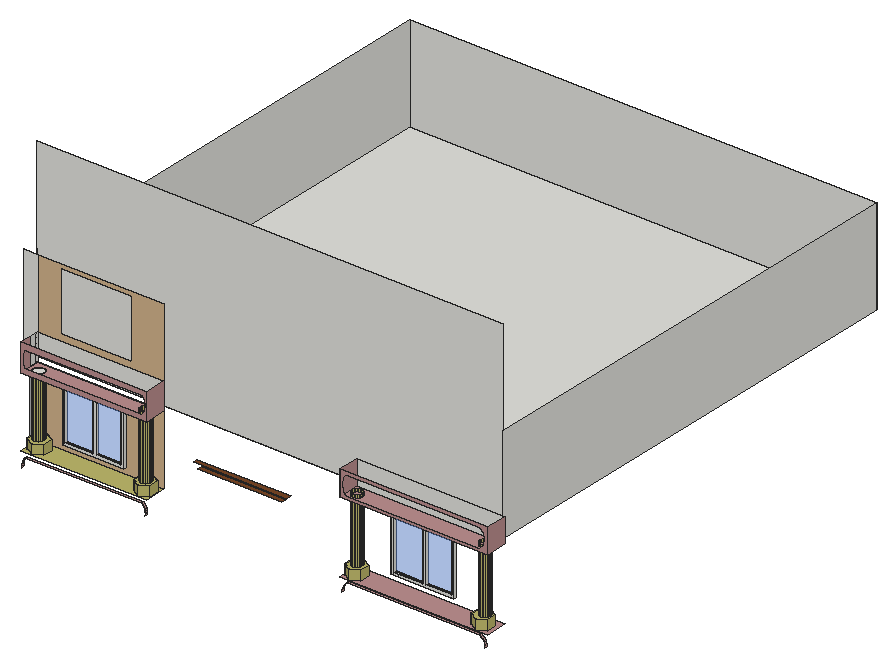
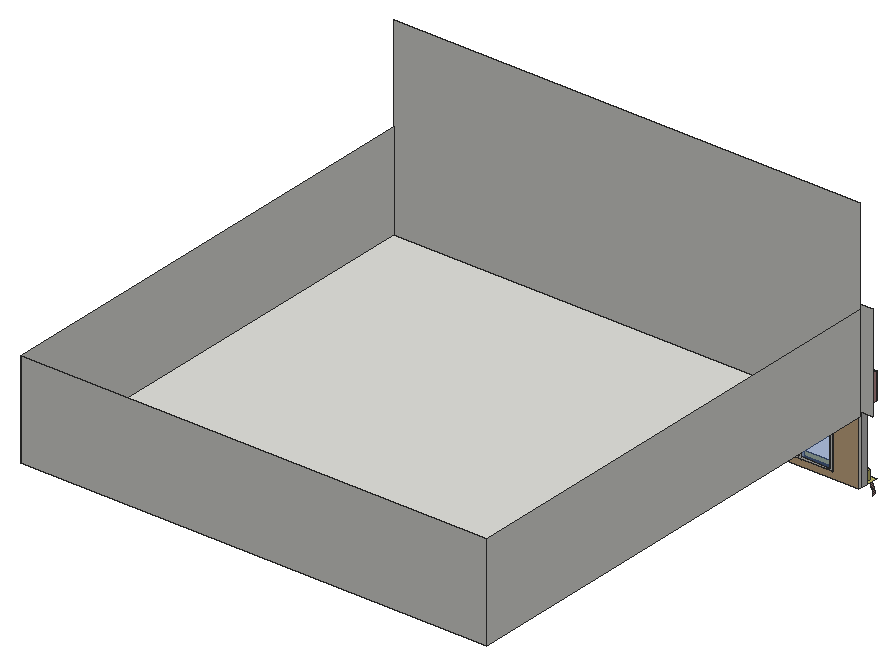
# SketchUp Ruby script. Lengths in inches.
U = 1.inch
M = Sketchup.active_model
def pt(a) = Geom::Point3d.new(a.map { |v| v * U })
def face(e, loops, mat)
  f = e.add_face(loops[0].map { |a| pt(a) })
  loops[1..].each { |l| e.add_face(l.map { |a| pt(a) }).erase! }
  f.material = f.back_material = mat if mat
  f
end
# faces: each face lists its corners as indices into pts; further lists are holes
def faces(e, pts, list, mat = nil) = list.each { |f| face(e, (f[0].is_a?(Array) ? f : [f]).map { |l| l.map { |i| pts[i] } }, mat) }
# xy, xz, yz: faces in a plane at the given z, y or x. An outline is a flat list of corners, or four numbers for a rectangle; further outlines are holes
def ring(l) = l.size == 4 ? [[l[0], l[1]], [l[2], l[1]], [l[2], l[3]], [l[0], l[3]]] : l.each_slice(2).to_a
def flat(e, list, mat, &to3) = list.each { |f| face(e, (f[0].is_a?(Array) ? f : [f]).map { |l| ring(l).map { |u, v| to3.(u, v) } }, mat) }
def xy(e, z, list, mat = nil) = flat(e, list, mat) { |x, y| [x, y, z] }
def xz(e, y, list, mat = nil) = flat(e, list, mat) { |x, z| [x, y, z] }
def yz(e, x, list, mat = nil) = flat(e, list, mat) { |y, z| [x, y, z] }
def lines(e, pts, list) = list.each { |a, b| e.add_line(pt(pts[a]), pt(pts[b])) }
# prism: a flat outline (further loops are holes) pulled along v
def prism(e, loops, v, mat = nil)
  f = face(e, loops, mat); d = Geom::Vector3d.new(v.map { |x| x * U })
  f.pushpull(f.normal.samedirection?(d) ? d.length : -d.length)
end
def box(e, o, s, mat = nil) = prism(e, [[o, [o[0] + s[0], o[1], o[2]], [o[0] + s[0], o[1] + s[1], o[2]], [o[0], o[1] + s[1], o[2]]]], [0, 0, s[2]], mat)
def at(x, y, z, deg = 0) = Geom::Transformation.translation(pt([x, y, z])) * Geom::Transformation.rotation(ORIGIN, Z_AXIS, deg.degrees)
def axes(o, x, y, z) = Geom::Transformation.new([*x, 0, *y, 0, *z, 0, *pt(o).to_a, 1])
def part(name) = M.definitions.add(name)
# library, detail: a bought-in or finely detailed component or shape, given as its bounding box
def library(name, o, s) = part(name).tap { |d| box(d.entities, o, s) }
def detail(e, o, s) = box(e.add_group.entities, o, s)
def put(e, d, t, mat = nil) = e.add_instance(d, t).tap { |i| i.material = mat if mat }
def group(e, t, mat = nil) = e.add_group.tap { |g| g.transformation = t; g.material = mat if mat }.entities
root = M.entities
M.materials.add("[0035_Tan]").color = [210, 180, 140]
M.materials.add("[0057_DarkKhaki]").color = [189, 183, 107]
M.materials.add("[0119_RosyBrown]").color = [188, 143, 143]
M.materials.add("[0131_Silver]").color = [192, 192, 192]
M.materials.add("[Translucent Glass Blue]").color = [100, 149, 237]
M.materials["[Translucent Glass Blue]"].alpha = 0.5
M.materials.add("[Wood Veneer 01]").color = [120, 70, 37]
xy(root,266.92,[[148.32,89.37,293.79,92.37]],"[0119_RosyBrown]")
xy(root,268.25,[[550.92,89.37,715.74,92.37]],"[0119_RosyBrown]")
xy(root,271.25,[[[540.59,89.37,725.37,116.37],[551.8,90.48,541.51,96.42,541.51,108.29,551.8,114.23,562.08,108.29,562.08,96.42],[709.73,90.48,699.45,96.42,699.45,108.29,709.73,114.23,720.02,108.29,720.02,96.42]]],"[0119_RosyBrown]")
xy(root,272.875,[[[142.36,89.37,299.74,116.37],[288.3125,90.3,277.98,96.26,277.98,108.2,288.3125,114.17,298.65,108.2,298.65,96.26],[155.8125,90.3,145.48,96.26,145.48,108.2,155.8125,114.17,166.15,108.2,166.15,96.26]]],"[0057_DarkKhaki]")
xy(root,279.75,[[586.09,113.37,664.21,116.37]])
xy(root,280.42,[[175.65,113.37,252.02,116.37]])
xy(root,282.75,[[589.09,113.37,625.15,116.37],[628.82,113.37,661.21,116.37]])
xy(root,283.25,[[[551.8,90.48,562.08,96.42,562.08,108.29,551.8,114.23,541.51,108.29,541.51,96.42],[551.49,97.26,549.85,97.47,548.33,98.1,547.02,99.11,546.02,100.41,545.39,101.9375,545.17,103.57,545.39,105.2,546.02,106.73,547.02,108.03,548.33,109.04,549.85,109.67,551.49,109.88,553.12,109.67,554.64,109.04,555.95,108.03,556.95,106.73,557.58,105.2,557.8,103.57,557.58,101.9375,556.95,100.41,555.95,99.11,554.64,98.1,553.12,97.47]],[[709.73,90.48,720.02,96.42,720.02,108.29,709.73,114.23,699.45,108.29,699.45,96.42],[711.11,97.26,709.48,97.47,707.95,98.1,706.65,99.11,705.64,100.41,705.01,101.9375,704.8,103.57,705.01,105.2,705.64,106.73,706.65,108.03,707.95,109.04,709.48,109.67,711.11,109.88,712.74,109.67,714.27,109.04,715.57,108.03,716.58,106.73,717.21,105.2,717.42,103.57,717.21,101.9375,716.58,100.41,715.57,99.11,714.27,98.1,712.74,97.47]]],"[0057_DarkKhaki]")
xy(root,283.42,[[178.65,113.37,213.84,116.37],[218.03,113.37,249.02,116.37]])
xy(root,284.875,[[[155.8125,90.3,166.15,96.26,166.15,108.2,155.8125,114.17,145.48,108.2,145.48,96.26],[153.85,96.4,152.14,96.77,150.59,97.57,149.3,98.75,148.36,100.22,147.83,101.88,147.74,103.62,148.11,105.33,148.91,106.88,150.09,108.17,151.56,109.11,153.22,109.65,154.96,109.73,156.67,109.36,158.22,108.56,159.51,107.38,160.46,105.91,160.99,104.25,161.07,102.51,160.7,100.8,159.9,99.25,158.72,97.96,157.26,97.01,155.59,96.48]],[[288.3125,90.3,298.65,96.26,298.65,108.2,288.3125,114.17,277.98,108.2,277.98,96.26],[287.6,96.4,285.89,96.77,284.34,97.57,283.05,98.75,282.11,100.22,281.58,101.88,281.49,103.62,281.86,105.33,282.66,106.88,283.84,108.17,285.31,109.11,286.97,109.65,288.71,109.73,290.42,109.36,291.97,108.56,293.26,107.38,294.21,105.91,294.74,104.25,294.82,102.51,294.45,100.8,293.65,99.25,292.47,97.96,291.01,97.01,289.34,96.48]]],"[0057_DarkKhaki]")
xy(root,340.81,[[376.4,74.37,481.09,80.37]],"[Wood Veneer 01]")
xy(root,346.81,[[370.4,74.37,487.09,80.37]],"[Wood Veneer 01]")
xy(root,351.13,[[589.09,113.37,625.15,116.37],[628.82,113.37,661.21,116.37]])
xy(root,353.8,[[178.65,113.37,213.84,116.37],[218.03,113.37,249.02,116.37]])
xy(root,354.13,[[586.09,113.37,664.21,116.37]])
xy(root,356.8,[[175.65,113.37,252.02,116.37]])
xy(root,360,[[153.85,96.4,155.59,96.48,157.26,97.01,158.72,97.96,159.9,99.25,160.7,100.8,161.07,102.51,160.99,104.25,160.46,105.91,159.51,107.38,158.22,108.56,156.67,109.36,154.96,109.73,153.22,109.65,151.56,109.11,150.09,108.17,148.91,106.88,148.11,105.33,147.74,103.62,147.83,101.88,148.36,100.22,149.3,98.75,150.59,97.57,152.14,96.77],[134.37,125.37,716.37,707.37]])
xy(root,360,[[142.36,89.37,299.68,116.37]],"[0119_RosyBrown]")
xy(root,361,[[540.59,89.37,725.37,116.37]],"[0119_RosyBrown]")
xz(root,89.37,[[[142.36,360,299.68,393.6875],[148.36,366,147.34,367.63,146.48,369.35,145.81,371.16,145.32,373.02,145.03,374.92,144.93,376.84,145.03,378.77,145.32,380.67,145.81,382.53,146.48,384.33,147.34,386.06,148.36,387.6875,293.68,387.6875,295.15,386.26,296.41,384.625,297.41,382.83,298.14,380.9,298.59,378.9,298.74,376.84,298.59,374.79,298.14,372.78,297.41,370.86,296.41,369.0625,295.15,367.43,293.68,366]],[[540.59,361,725.37,391.75],[549.67,364,547.9,365.59,546.4,367.43,545.19,369.48,544.3125,371.6875,543.77,374,543.59,376.375,543.77,378.75,544.3125,381.0625,545.19,383.27,546.4,385.32,547.9,387.16,549.67,388.75,714.61,388.75,716.81,387.42,718.71,385.71,720.27,383.68,721.42,381.39,722.13,378.93,722.37,376.375,722.13,373.82,721.42,371.36,720.27,369.07,718.71,367.04,716.81,365.33,714.61,364]]],"[0119_RosyBrown]")
xz(root,113.37,[[[586.09,279.75,664.21,354.13],[589.09,282.75,625.15,351.13],[628.82,282.75,661.21,351.13]],[[175.65,280.42,252.02,356.8],[178.65,283.42,213.84,353.8],[218.03,283.42,249.02,353.8]]])
xz(root,116.37,[[[586.09,279.75,664.21,354.13],[589.09,282.75,625.15,351.13],[628.82,282.75,661.21,351.13]],[[175.65,280.42,252.02,356.8],[178.65,283.42,213.84,353.8],[218.03,283.42,249.02,353.8]],[125.37,360,142.36,480],[540.59,361,725.37,391.75]])
xz(root,116.37,[[[142.36,272.875,299.74,360],[175.65,280.42,252.02,356.8]],[[299.68,360,299.74,360,299.74,480,142.36,480,142.36,393.6875,299.68,393.6875],[170.78,401.45,260.03,475.13]]],"[0035_Tan]")
xz(root,116.37,[[589.09,282.75,625.15,351.13],[628.82,282.75,661.21,351.13],[178.65,283.42,213.84,353.8],[218.03,283.42,249.02,353.8]],"[Translucent Glass Blue]")
xz(root,125.37,[[134.37,360,716.37,600]])
xz(root,707.37,[[134.37,360,716.37,480]])
yz(root,134.37,[[125.37,360,707.37,480]])
yz(root,142.36,[[113.37,272.875,116.37,360],[104.37,360,113.37,393.6875],[113.37,360,116.37,393.6875]])
yz(root,142.36,[[89.37,360,104.37,393.6875]],"[0119_RosyBrown]")
yz(root,142.36,[[104.37,272.875,113.37,360]],"[0131_Silver]")
yz(root,145.48,[[96.26,272.875,108.2,284.875]],"[0057_DarkKhaki]")
yz(root,166.15,[[96.26,272.875,108.2,284.875]],"[0057_DarkKhaki]")
yz(root,175.65,[[113.37,280.42,116.37,356.8]])
yz(root,178.65,[[113.37,283.42,116.37,353.8]])
yz(root,213.84,[[113.37,283.42,116.37,353.8]])
yz(root,218.03,[[113.37,283.42,116.37,353.8]])
yz(root,249.02,[[113.37,283.42,116.37,353.8]])
yz(root,252.02,[[113.37,280.42,116.37,356.8]])
yz(root,277.98,[[96.26,272.875,108.2,284.875]],"[0057_DarkKhaki]")
yz(root,298.65,[[96.26,272.875,108.2,284.875]],"[0057_DarkKhaki]")
yz(root,299.68,[[89.37,360,116.37,393.6875]],"[0119_RosyBrown]")
yz(root,540.59,[[89.37,361,116.37,391.75]],"[0119_RosyBrown]")
yz(root,541.51,[[96.42,271.25,108.29,283.25]],"[0057_DarkKhaki]")
yz(root,562.08,[[96.42,271.25,108.29,283.25]],"[0057_DarkKhaki]")
yz(root,586.09,[[113.37,279.75,116.37,354.13]])
yz(root,589.09,[[113.37,282.75,116.37,351.13]])
yz(root,625.15,[[113.37,282.75,116.37,351.13]])
yz(root,628.82,[[113.37,282.75,116.37,351.13]])
yz(root,661.21,[[113.37,282.75,116.37,351.13]])
yz(root,664.21,[[113.37,279.75,116.37,354.13]])
yz(root,699.45,[[96.42,271.25,108.29,283.25]],"[0057_DarkKhaki]")
yz(root,716.37,[[125.37,360,707.37,480]])
yz(root,720.02,[[96.42,271.25,108.29,283.25]],"[0057_DarkKhaki]")
yz(root,725.37,[[89.37,361,116.37,391.75]],"[0119_RosyBrown]")
p = [[144.55,92.37,254.54],[144.44,92.37,256.4375],[144.44,89.37,256.4375],[144.55,89.37,254.54],[298.47,92.37,256.4375],[298.34,92.37,254.47],
  [298.34,89.37,254.47],[298.47,89.37,256.4375],[543.59,92.37,255.875],[543.82,92.37,258.375],[543.82,89.37,258.375],[543.59,89.37,255.875],
  [722.17,92.37,258.3],[722.37,92.37,255.875],[722.37,89.37,255.875],[722.17,89.37,258.3],[144.55,92.37,258.34],[144.55,89.37,258.34],
  [298.34,92.37,258.4],[298.34,89.37,258.4],[144.89,92.37,260.21],[144.89,89.37,260.21],[721.58,92.37,260.66],[721.58,89.37,260.66],
  [297.93,92.37,260.33],[297.93,89.37,260.33],[544.48,92.37,260.8],[544.48,89.37,260.8],[145.44,92.37,262.03],[145.44,89.37,262.03],
  [297.25,92.37,262.18],[297.25,89.37,262.18],[720.6,92.37,262.9],[720.6,89.37,262.9],[545.5625,92.37,263.06],[545.5625,89.37,263.06],
  [146.21,92.37,263.77],[146.21,89.37,263.77],[296.32,92.37,263.92],[296.32,89.37,263.92],[719.28,92.37,264.9375],[719.28,89.37,264.9375],
  [547.03,92.37,265.1],[547.03,89.37,265.1],[147.17,92.37,265.41],[147.17,89.37,265.41],[295.16,92.37,265.51],[295.16,89.37,265.51],
  [717.65,92.37,266.74],[717.65,89.37,266.74],[548.83,92.37,266.85],[548.83,89.37,266.85],[148.32,92.37,266.92],[148.32,89.37,266.92],
  [293.79,92.37,266.92],[293.79,89.37,266.92],[715.74,92.37,268.25],[715.74,89.37,268.25],[550.92,92.37,268.25],[550.92,89.37,268.25],
  [541.51,96.42,271.25],[551.8,90.48,271.25],[551.8,90.48,283.25],[541.51,96.42,283.25],[562.08,96.42,271.25],[562.08,96.42,283.25],
  [699.45,96.42,271.25],[709.73,90.48,271.25],[709.73,90.48,283.25],[699.45,96.42,283.25],[720.02,96.42,271.25],[720.02,96.42,283.25],
  [551.8,114.23,271.25],[541.51,108.29,271.25],[541.51,108.29,283.25],[551.8,114.23,283.25],[562.08,108.29,271.25],[562.08,108.29,283.25],
  [709.73,114.23,271.25],[699.45,108.29,271.25],[699.45,108.29,283.25],[709.73,114.23,283.25],[720.02,108.29,271.25],[720.02,108.29,283.25],
  [145.48,96.26,272.875],[155.8125,90.3,272.875],[155.8125,90.3,284.875],[145.48,96.26,284.875],[166.15,96.26,272.875],[166.15,96.26,284.875],
  [277.98,96.26,272.875],[288.3125,90.3,272.875],[288.3125,90.3,284.875],[277.98,96.26,284.875],[298.65,96.26,272.875],[298.65,96.26,284.875],
  [155.8125,114.17,272.875],[145.48,108.2,272.875],[145.48,108.2,284.875],[155.8125,114.17,284.875],[166.15,108.2,272.875],[166.15,108.2,284.875],
  [288.3125,114.17,272.875],[277.98,108.2,272.875],[277.98,108.2,284.875],[288.3125,114.17,284.875],[298.65,108.2,272.875],[298.65,108.2,284.875],
  [549.85,97.47,283.25],[551.49,97.26,283.25],[551.49,97.26,364],[549.85,97.47,364],[553.12,97.47,283.25],[553.12,97.47,364],
  [709.48,97.47,283.25],[711.11,97.26,283.25],[711.11,97.26,364],[709.48,97.47,364],[712.74,97.47,283.25],[712.74,97.47,364],
  [548.33,98.1,283.25],[548.33,98.1,364],[554.64,98.1,283.25],[554.64,98.1,364],[707.95,98.1,283.25],[707.95,98.1,364],
  [714.27,98.1,283.25],[714.27,98.1,364],[547.02,99.11,283.25],[547.02,99.11,364],[555.95,99.11,283.25],[555.95,99.11,364],
  [706.65,99.11,283.25],[706.65,99.11,364],[715.57,99.11,283.25],[715.57,99.11,364],[546.02,100.41,283.25],[546.02,100.41,364],
  [556.95,100.41,283.25],[556.95,100.41,364],[705.64,100.41,283.25],[705.64,100.41,364],[716.58,100.41,283.25],[716.58,100.41,364],
  [545.39,101.9375,283.25],[545.39,101.9375,364],[557.58,101.9375,283.25],[557.58,101.9375,364],[705.01,101.9375,283.25],[705.01,101.9375,364],
  [717.21,101.9375,283.25],[717.21,101.9375,364],[545.17,103.57,283.25],[545.17,103.57,364],[557.8,103.57,283.25],[557.8,103.57,364],
  [704.8,103.57,283.25],[704.8,103.57,364],[717.42,103.57,283.25],[717.42,103.57,364],[545.39,105.2,283.25],[545.39,105.2,364],
  [557.58,105.2,283.25],[557.58,105.2,364],[705.01,105.2,283.25],[705.01,105.2,364],[717.21,105.2,283.25],[717.21,105.2,364],
  [546.02,106.73,283.25],[546.02,106.73,364],[556.95,106.73,283.25],[556.95,106.73,364],[705.64,106.73,283.25],[705.64,106.73,364],
  [716.58,106.73,283.25],[716.58,106.73,364],[547.02,108.03,283.25],[547.02,108.03,364],[555.95,108.03,283.25],[555.95,108.03,364],
  [706.65,108.03,283.25],[706.65,108.03,364],[715.57,108.03,283.25],[715.57,108.03,364],[548.33,109.04,283.25],[548.33,109.04,364],
  [554.64,109.04,283.25],[554.64,109.04,364],[707.95,109.04,283.25],[707.95,109.04,364],[714.27,109.04,283.25],[714.27,109.04,364],
  [549.85,109.67,283.25],[549.85,109.67,364],[553.12,109.67,283.25],[553.12,109.67,364],[709.48,109.67,283.25],[709.48,109.67,364],
  [712.74,109.67,283.25],[712.74,109.67,364],[551.49,109.88,283.25],[551.49,109.88,364],[711.11,109.88,283.25],[711.11,109.88,364],
  [152.14,96.77,284.875],[153.85,96.4,284.875],[153.85,96.4,360],[152.14,96.77,360],[155.59,96.48,284.875],[155.59,96.48,360],
  [285.89,96.77,284.875],[287.6,96.4,284.875],[287.6,96.4,364.25],[285.89,96.77,364.25],[289.34,96.48,284.875],[289.34,96.48,364.25],
  [157.26,97.01,284.875],[157.26,97.01,360],[291.01,97.01,284.875],[291.01,97.01,364.25],[150.59,97.57,284.875],[150.59,97.57,360],
  [284.34,97.57,284.875],[284.34,97.57,364.25],[158.72,97.96,284.875],[158.72,97.96,360],[292.47,97.96,284.875],[292.47,97.96,364.25],
  [149.3,98.75,284.875],[149.3,98.75,360],[283.05,98.75,284.875],[283.05,98.75,364.25],[159.9,99.25,284.875],[159.9,99.25,360],
  [293.65,99.25,284.875],[293.65,99.25,364.25],[148.36,100.22,284.875],[148.36,100.22,360],[282.11,100.22,284.875],[282.11,100.22,364.25],
  [160.7,100.8,284.875],[160.7,100.8,360],[294.45,100.8,284.875],[294.45,100.8,364.25],[147.83,101.88,284.875],[147.83,101.88,360],
  [281.58,101.88,284.875],[281.58,101.88,364.25],[161.07,102.51,284.875],[161.07,102.51,360],[294.82,102.51,284.875],[294.82,102.51,364.25],
  [147.74,103.62,284.875],[147.74,103.62,360],[281.49,103.62,284.875],[281.49,103.62,364.25],[160.99,104.25,284.875],[160.99,104.25,360],
  [294.74,104.25,284.875],[294.74,104.25,364.25],[148.11,105.33,284.875],[148.11,105.33,360],[281.86,105.33,284.875],[281.86,105.33,364.25],
  [160.46,105.91,284.875],[160.46,105.91,360],[294.21,105.91,284.875],[294.21,105.91,364.25],[148.91,106.88,284.875],[148.91,106.88,360],
  [282.66,106.88,284.875],[282.66,106.88,364.25],[159.51,107.38,284.875],[159.51,107.38,360],[293.26,107.38,284.875],[293.26,107.38,364.25],
  [150.09,108.17,284.875],[150.09,108.17,360],[283.84,108.17,284.875],[283.84,108.17,364.25],[158.22,108.56,284.875],[158.22,108.56,360],
  [291.97,108.56,284.875],[291.97,108.56,364.25],[151.56,109.11,284.875],[151.56,109.11,360],[285.31,109.11,284.875],[285.31,109.11,364.25],
  [156.67,109.36,284.875],[156.67,109.36,360],[290.42,109.36,284.875],[290.42,109.36,364.25],[153.22,109.65,284.875],[153.22,109.65,360],
  [286.97,109.65,284.875],[286.97,109.65,364.25],[154.96,109.73,284.875],[154.96,109.73,360],[288.71,109.73,284.875],[288.71,109.73,364.25]]
faces(root,p,[[0,1,2,3],[4,5,6,7],[8,9,10,11],[12,13,14,15],[1,16,17,2],[18,4,7,19],[16,20,21,17],[22,12,15,23],
  [24,18,19,25],[9,26,27,10],[20,28,29,21],[30,24,25,31],[32,22,23,33],[26,34,35,27],[28,36,37,29],[38,30,31,39],
  [40,32,33,41],[34,42,43,35],[36,44,45,37],[46,38,39,47],[48,40,41,49],[42,50,51,43],[44,52,53,45],[54,46,47,55],
  [56,48,49,57],[50,58,59,51]],"[0119_RosyBrown]")
faces(root,p,[[60,61,62,63],[61,64,65,62],[66,67,68,69],[67,70,71,68],[76,72,75,77],[84,85,86,87],[85,88,89,86],[90,91,92,93],
  [91,94,95,92],[108,109,110,111],[109,112,113,110],[114,115,116,117],[115,118,119,116],[120,108,111,121],[112,122,123,113],[124,114,117,125],
  [118,126,127,119],[128,120,121,129],[122,130,131,123],[132,124,125,133],[126,134,135,127],[136,128,129,137],[130,138,139,131],[140,132,133,141],
  [134,142,143,135],[144,136,137,145],[138,146,147,139],[148,140,141,149],[142,150,151,143],[152,144,145,153],[146,154,155,147],[156,148,149,157],
  [150,158,159,151],[160,152,153,161],[154,162,163,155],[164,156,157,165],[158,166,167,159],[168,160,161,169],[162,170,171,163],[172,164,165,173],
  [166,174,175,167],[176,168,169,177],[170,178,179,171],[180,172,173,181],[174,182,183,175],[184,176,177,185],[178,186,187,179],[188,180,181,189],
  [182,190,191,183],[192,184,185,193],[186,194,195,187],[196,188,189,197],[190,198,199,191],[200,192,193,201],[194,200,201,195],[202,196,197,203],
  [198,202,203,199],[204,205,206,207],[205,208,209,206],[210,211,212,213],[211,214,215,212],[208,216,217,209],[214,218,219,215],[220,204,207,221],
  [222,210,213,223],[216,224,225,217],[218,226,227,219],[228,220,221,229],[230,222,223,231],[224,232,233,225],[226,234,235,227],[236,228,229,237],
  [238,230,231,239],[232,240,241,233],[234,242,243,235],[244,236,237,245],[246,238,239,247],[240,248,249,241],[242,250,251,243],[252,244,245,253],
  [254,246,247,255],[248,256,257,249],[250,258,259,251],[260,252,253,261],[262,254,255,263],[256,264,265,257],[258,266,267,259],[268,260,261,269],
  [270,262,263,271],[264,272,273,265],[266,274,275,267],[276,268,269,277],[278,270,271,279],[272,280,281,273],[274,282,283,275],[284,276,277,285],
  [286,278,279,287],[280,288,289,281],[282,290,291,283],[292,284,285,293],[294,286,287,295],[288,296,297,289],[290,298,299,291],[296,292,293,297],
  [298,294,295,299]],"[0057_DarkKhaki]")
faces(root,p,[[72,73,74,75],[78,79,80,81],[82,78,81,83],[96,97,98,99],[100,96,99,101],[102,103,104,105],[106,102,105,107]])
